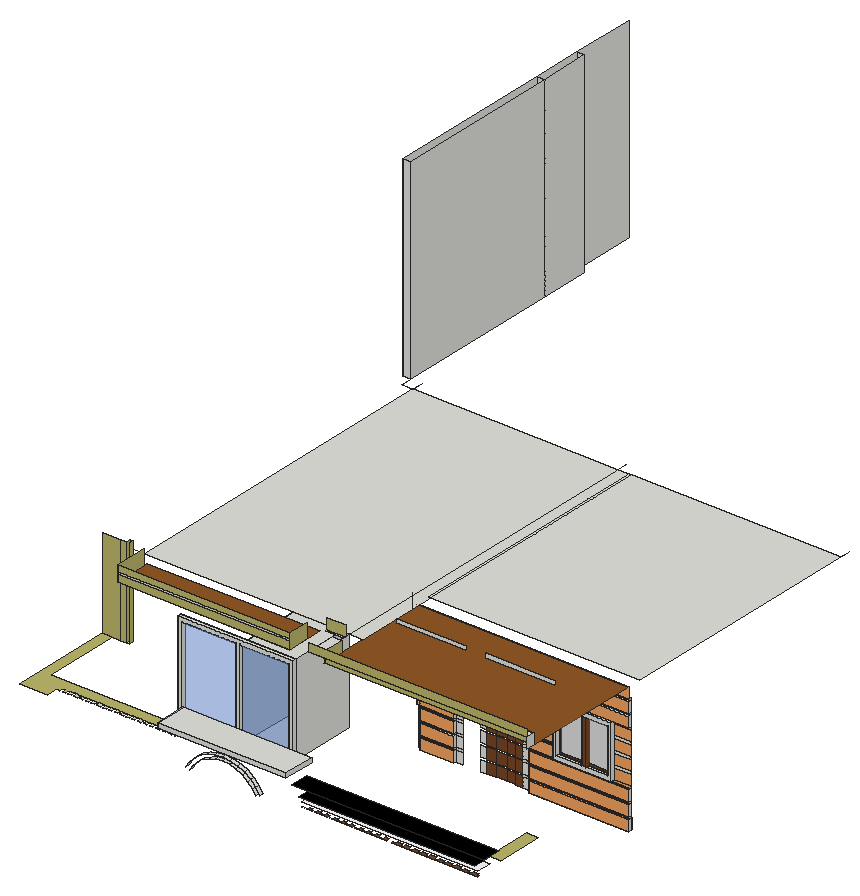
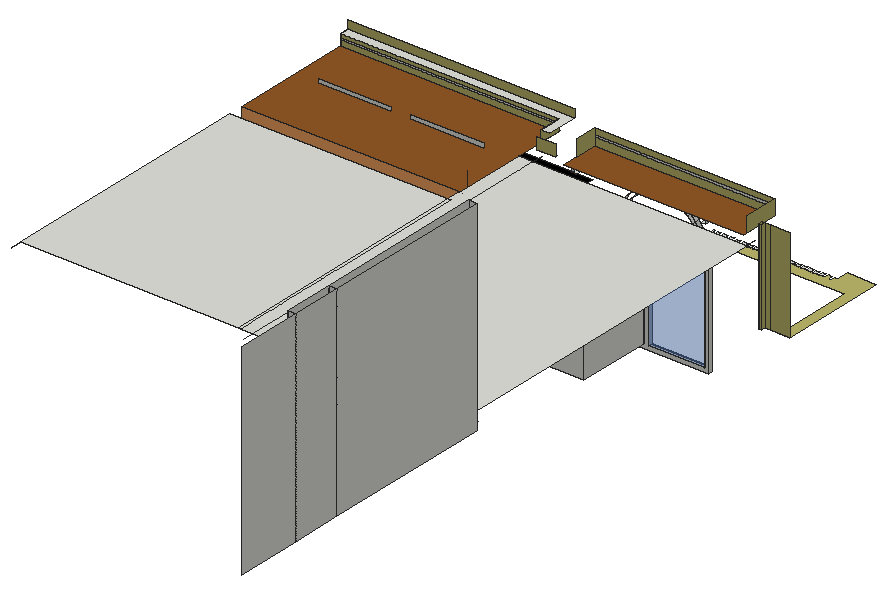
# SketchUp Ruby script. Lengths in inches.
U = 1.inch
M = Sketchup.active_model
def pt(a) = Geom::Point3d.new(a.map { |v| v * U })
def face(e, loops, mat)
  f = e.add_face(loops[0].map { |a| pt(a) })
  loops[1..].each { |l| e.add_face(l.map { |a| pt(a) }).erase! }
  f.material = f.back_material = mat if mat
  f
end
# faces: each face lists its corners as indices into pts; further lists are holes
def faces(e, pts, list, mat = nil) = list.each { |f| face(e, (f[0].is_a?(Array) ? f : [f]).map { |l| l.map { |i| pts[i] } }, mat) }
# xy, xz, yz: faces in a plane at the given z, y or x. An outline is a flat list of corners, or four numbers for a rectangle; further outlines are holes
def ring(l) = l.size == 4 ? [[l[0], l[1]], [l[2], l[1]], [l[2], l[3]], [l[0], l[3]]] : l.each_slice(2).to_a
def flat(e, list, mat, &to3) = list.each { |f| face(e, (f[0].is_a?(Array) ? f : [f]).map { |l| ring(l).map { |u, v| to3.(u, v) } }, mat) }
def xy(e, z, list, mat = nil) = flat(e, list, mat) { |x, y| [x, y, z] }
def xz(e, y, list, mat = nil) = flat(e, list, mat) { |x, z| [x, y, z] }
def yz(e, x, list, mat = nil) = flat(e, list, mat) { |y, z| [x, y, z] }
def lines(e, pts, list) = list.each { |a, b| e.add_line(pt(pts[a]), pt(pts[b])) }
# prism: a flat outline (further loops are holes) pulled along v
def prism(e, loops, v, mat = nil)
  f = face(e, loops, mat); d = Geom::Vector3d.new(v.map { |x| x * U })
  f.pushpull(f.normal.samedirection?(d) ? d.length : -d.length)
end
def box(e, o, s, mat = nil) = prism(e, [[o, [o[0] + s[0], o[1], o[2]], [o[0] + s[0], o[1] + s[1], o[2]], [o[0], o[1] + s[1], o[2]]]], [0, 0, s[2]], mat)
def at(x, y, z, deg = 0) = Geom::Transformation.translation(pt([x, y, z])) * Geom::Transformation.rotation(ORIGIN, Z_AXIS, deg.degrees)
def axes(o, x, y, z) = Geom::Transformation.new([*x, 0, *y, 0, *z, 0, *pt(o).to_a, 1])
def part(name) = M.definitions.add(name)
# library, detail: a bought-in or finely detailed component or shape, given as its bounding box
def library(name, o, s) = part(name).tap { |d| box(d.entities, o, s) }
def detail(e, o, s) = box(e.add_group.entities, o, s)
def put(e, d, t, mat = nil) = e.add_instance(d, t).tap { |i| i.material = mat if mat }
def group(e, t, mat = nil) = e.add_group.tap { |g| g.transformation = t; g.material = mat if mat }.entities
root = M.entities
M.materials.add("[0010_Snow]").color = [255, 250, 250]
M.materials.add("[0037_SandyBrown]").color = [244, 164, 96]
M.materials.add("[0057_DarkKhaki]").color = [189, 183, 107]
M.materials.add("[0137_Black]").color = [0, 0, 0]
M.materials.add("[Translucent Glass Blue]").color = [100, 149, 237]
M.materials["[Translucent Glass Blue]"].alpha = 0.5
M.materials.add("[Translucent Glass Gray]").color = [128, 128, 128]
M.materials["[Translucent Glass Gray]"].alpha = 0.5
M.materials.add("[Wood Floor Parquet]").color = [145, 89, 39]
M.materials.add("[Wood Veneer 01]").color = [120, 70, 37]
xy(root,15.35,[[88.6875,87.625,180.5,90.625]])
xy(root,16.53,[[227.125,155.75,254.53,157.75],[314.53,155.75,394.3125,157.75],[314.53,157.75,394.3125,158.9375]])
xy(root,18.35,[[91.6875,87.625,134.59,90.625],[138.39,87.625,177.5,90.625],[138.39,90.625,177.5,147.4375]])
xy(root,24.9375,[[314.53,157.75,394.3125,158.9375]])
xy(root,24.9375,[[227.125,155.75,254.53,157.75],[314.53,155.75,394.3125,157.75]],"[0037_SandyBrown]")
xy(root,27.1,[[227.125,155.75,254.53,157.75],[314.53,155.75,394.3125,157.75]])
xy(root,35.5,[[227.125,155.75,254.53,157.75]])
xy(root,35.5,[[314.53,155.75,394.3125,157.75]],"[0037_SandyBrown]")
xy(root,37.66,[[227.125,155.75,254.53,157.75],[314.53,155.75,394.3125,157.75]])
xy(root,44.24,[[246.54,13.8125,246.54,14.8125,250.6,14.8125,250.6,16.8125,253.29,16.8125,253.29,14.8125,257.35,14.8125,257.35,16.8125,260.04,16.8125,260.04,14.8125,264.1,14.8125,264.1,16.8125,266.79,16.8125,266.79,14.8125,270.85,14.8125,270.85,16.8125,273.54,16.8125,273.54,14.8125,277.6,14.8125,277.6,16.8125,280.29,16.8125,280.29,14.8125,284.35,14.8125,284.35,16.8125,287.04,16.8125,287.04,14.8125,291.1,14.8125,291.1,16.8125,293.79,16.8125,293.79,14.8125,297.85,14.8125,297.85,16.8125,300.54,16.8125,300.54,14.8125,304.6,14.8125,304.6,16.8125,307.29,16.8125,307.29,14.8125,311.35,14.8125,311.35,16.8125,314.04,16.8125,314.04,14.8125,314.71,14.8125,314.71,13.8125],[318.91,13.8125,318.91,14.8125,320.79,14.8125,320.79,16.8125,324.85,16.8125,324.85,14.8125,327.54,14.8125,327.54,16.8125,331.6,16.8125,331.6,14.8125,334.29,14.8125,334.29,16.8125,338.35,16.8125,338.35,14.8125,341.04,14.8125,341.04,16.8125,345.1,16.8125,345.1,14.8125,347.79,14.8125,347.79,16.8125,351.85,16.8125,351.85,14.8125,354.54,14.8125,354.54,16.8125,358.6,16.8125,358.6,14.8125,361.29,14.8125,361.29,16.8125,365.35,16.8125,365.35,14.8125,368.04,14.8125,368.04,16.8125,372.1,16.8125,372.1,14.8125,374.79,14.8125,374.79,16.8125,378.85,16.8125,378.85,14.8125,381.54,14.8125,381.54,16.8125,385.6,16.8125,385.6,14.8125,387.24,14.8125,387.24,13.8125]],"[Wood Veneer 01]")
xy(root,46.0625,[[227.125,155.75,254.53,157.75],[314.53,155.75,394.3125,157.75]])
xy(root,48.04,[[334.36,154.75,381.24,157.75]])
xy(root,48.11,[[246.54,13.8125,387.24,25.8125]],"[0010_Snow]")
xy(root,48.22,[[225.0625,155.75,227.125,157.75],[227.125,155.75,254.53,157.75],[314.53,155.75,334.36,157.75]])
xy(root,51.04,[[337.36,154.75,357.8,157.75],[360.74,154.75,378.24,157.75]])
xy(root,53.24,[[246.54,10.8125,387.24,25.8125]],"[0137_Black]")
xy(root,56.625,[[225.0625,155.75,227.125,157.75],[227.125,155.75,254.53,157.75],[314.53,155.75,334.36,157.75]])
xy(root,58.78,[[225.0625,155.75,227.125,157.75],[227.125,155.75,254.53,157.75],[314.53,155.75,334.36,157.75]])
xy(root,60,[[59.94,13.8125,62.74,16.8125],[64.57,13.8125,67.37,16.8125],[69.19,13.8125,71.99,16.8125],[73.82,13.8125,76.62,16.8125],[78.44,13.8125,81.24,16.8125],
  [83.07,13.8125,85.87,16.8125],[87.69,13.8125,90.49,16.8125],[92.32,13.8125,95.12,16.8125],[96.94,13.8125,99.74,16.8125],[101.57,13.8125,104.37,16.8125],
  [106.19,13.8125,108.99,16.8125],[110.82,13.8125,113.62,16.8125],[115.44,13.8125,118.24,16.8125],[120.07,13.8125,122.87,16.8125],[125.13,13.8125,127.93,16.8125],
  [130.19,13.8125,132.99,16.8125],[135.25,13.8125,138.06,16.8125],[140.32,13.8125,143.12,16.8125],[145.38,13.8125,145.98,16.8125],[47.8125,87.625,50.0625,90.625]])
xy(root,60,[[28.5625,4.8125,50.69,4.8125,50.69,13.8125,53.49,13.8125,53.49,16.8125,55.32,16.8125,55.32,13.8125,58.12,13.8125,58.12,16.8125,145.98,16.8125,145.98,25.8125,36.25,25.8125,36.25,87.625,28.5625,87.625],[394.3125,16.8125,403.3125,54.1875]],"[0057_DarkKhaki]")
xy(root,60,[[241.27,10.8125,394.3125,25.8125]],"[0137_Black]")
xy(root,67.1875,[[225.0625,155.75,227.125,157.75],[227.125,155.75,254.53,157.75],[314.53,155.75,334.36,157.75]])
xy(root,69.35,[[225.0625,155.75,227.125,157.75],[227.125,155.75,254.53,157.75],[314.53,155.75,334.36,157.75],[225.0625,157.75,254.53,157.875]])
xy(root,70.61,[[142.42,0,142.42,25.8125,145.98,25.8125,145.98,4.8125,241.27,4.8125,241.27,25.8125,244.96,25.8125,244.96,0]])
xy(root,74.1875,[[142.42,0,244.96,25.8125]])
xy(root,77.75,[[225.0625,155.75,227.125,157.75],[314.53,155.75,334.36,157.75],[225.0625,157.75,254.53,157.875]])
xy(root,77.75,[[227.125,155.75,254.53,157.75]],"[0037_SandyBrown]")
xy(root,79.91,[[225.0625,155.75,227.125,157.75],[227.125,155.75,254.53,157.75],[314.53,155.75,334.36,157.75]])
xy(root,84,[[260.53,154.75,274.66,157.75],[274.66,154.75,279.73,157.75],[279.73,154.75,308.53,157.75]])
xy(root,87.22,[[337.36,154.75,357.8,157.75],[360.74,154.75,378.24,157.75]])
xy(root,88.3125,[[225.0625,155.75,227.125,157.75],[227.125,155.75,254.53,157.75],[314.53,155.75,334.36,157.75]])
xy(root,90,[[254.53,154.75,314.53,157.75]])
xy(root,90.22,[[334.36,154.75,381.24,157.75]])
xy(root,90.47,[[225.0625,155.75,227.125,157.75],[227.125,155.75,394.3125,157.75]])
xy(root,90.6,[[91.6875,87.625,134.59,90.625],[134.59,87.625,138.39,90.625],[138.39,87.625,177.5,90.625],[138.39,90.625,177.5,147.4375]])
xy(root,93.6,[[88.6875,87.625,180.5,90.625]])
xy(root,98.875,[[225.0625,155.75,227.125,157.75],[227.125,155.75,394.3125,157.75]])
xy(root,101.03,[[225.0625,155.75,227.125,157.75],[227.125,155.75,394.3125,157.75]])
xy(root,109.4375,[[225.0625,155.75,227.125,157.75],[227.125,155.75,394.3125,157.75]])
xy(root,111.6,[[225.0625,155.75,227.125,157.75],[227.125,155.75,394.3125,157.75]])
xy(root,120,[[52.3125,99.625,216.0625,367.8125],[216.0625,99.625,216.0625,367.8125,225.0625,367.8125,225.0625,166.75,227.125,166.75,227.125,99.625],[225.0625,166.75,227.125,367.8125],[227.125,166.75,394.3125,367.8125],[37.25,376.8125,43.3125,510.5],
  [37.25,510.5,43.3125,550.125]])
xy(root,120,[[61.7,61.0625,199.44,90.625],[227.125,61.0625,394.3125,155.75]],"[Wood Floor Parquet]")
xy(root,123.17,[[205.65,89.5625,220.06,90.625]])
xy(root,128.6875,[[220.06,54.1875,220.06,77.875,227.125,77.875,227.125,61.0625,394.3125,61.0625,394.3125,54.1875]])
xz(root,0,[[142.42,70.61,244.96,74.1875]])
xz(root,25.8125,[[241.27,70.61,244.96,70.75]])
xz(root,54.1875,[[220.06,128.6875,394.3125,134.75]],"[0057_DarkKhaki]")
xz(root,61.0625,[[227.125,124.34,394.3125,125.71],[61.7,126,199.44,127.5]])
xz(root,61.0625,[[61.7,120,199.44,126],[227.125,120,394.3125,124.34],[227.125,125.71,394.3125,128.6875],[61.7,127.5,199.44,132]],"[0057_DarkKhaki]")
xz(root,87.625,[[[88.6875,15.35,180.5,93.6],[91.6875,18.35,91.6875,90.6,177.5,90.6,177.5,18.35,138.39,18.35,138.39,90.6,134.59,90.6,134.59,18.35]]])
xz(root,87.625,[[28.5625,60,43.3125,132],[43.3125,60,47.8125,132]],"[0057_DarkKhaki]")
xz(root,90.625,[[[88.6875,15.35,180.5,93.6],[91.6875,18.35,134.59,18.35,134.59,90.6,138.39,90.6,138.39,18.35,177.5,18.35,177.5,90.6,91.6875,90.6]]])
xz(root,90.625,[[47.8125,60,50.0625,132],[205.65,123.17,220.06,132]],"[0057_DarkKhaki]")
xz(root,90.625,[[91.6875,18.35,134.59,90.6],[138.39,18.35,177.5,90.6]],"[Translucent Glass Blue]")
xz(root,116.875,[[239.99,129,295.56,132],[310.99,129,366.56,132]])
xz(root,147.4375,[[138.39,18.35,177.5,90.6]])
xz(root,154.75,[[[334.36,48.04,381.24,90.22],[337.36,51.04,378.24,87.22]]])
xz(root,154.75,[[357.8,51.04,360.74,87.22]],"[Wood Veneer 01]")
xz(root,155.75,[[225.0625,48.22,227.125,56.625],[225.0625,58.78,227.125,67.1875],[225.0625,69.35,227.125,77.75],[225.0625,79.91,227.125,88.3125],[225.0625,90.47,227.125,98.875],
  [225.0625,101.03,227.125,109.4375]])
xz(root,155.75,[[227.125,16.53,254.53,24.9375],[314.53,16.53,394.3125,24.9375],[227.125,27.1,254.53,35.5],[314.53,27.1,394.3125,35.5],[227.125,37.66,254.53,46.0625],
  [314.53,37.66,394.3125,46.0625],[227.125,48.22,254.53,56.625],[314.53,48.22,334.36,56.625],[227.125,58.78,254.53,67.1875],[314.53,58.78,334.36,67.1875],
  [227.125,69.35,254.53,77.75],[314.53,69.35,334.36,77.75],[227.125,79.91,254.53,88.3125],[314.53,79.91,334.36,88.3125],[227.125,90.47,394.3125,98.875],
  [227.125,101.03,394.3125,109.4375],[227.125,111.6,394.3125,120]],"[0037_SandyBrown]")
xz(root,157.75,[[225.0625,16.53,227.125,24.9375],[227.125,16.53,254.53,24.9375],[254.53,16.53,260.53,24.9375],[274.66,16.53,279.73,24.9375],[308.53,16.53,314.53,24.9375],
  [314.53,16.53,394.3125,24.9375],[225.0625,24.9375,227.125,27.1],[254.53,24.9375,260.53,27.1],[308.53,24.9375,314.53,27.1],[225.0625,27.1,227.125,35.5],
  [227.125,27.1,254.53,35.5],[254.53,27.1,260.53,35.5],[274.66,27.1,279.73,35.5],[308.53,27.1,314.53,35.5],[314.53,27.1,394.3125,35.5],
  [225.0625,35.5,227.125,37.66],[254.53,35.5,260.53,37.66],[308.53,35.5,314.53,37.66],[225.0625,37.66,227.125,46.0625],[254.53,37.66,260.53,46.0625],
  [274.66,37.66,279.73,46.0625],[308.53,37.66,314.53,46.0625],[314.53,37.66,394.3125,46.0625],[225.0625,46.0625,227.125,48.22],[254.53,46.0625,260.53,48.22],
  [308.53,46.0625,314.53,48.22],[334.36,48.04,381.24,48.22],[225.0625,48.22,254.53,56.625],[254.53,48.22,260.53,56.625],[274.66,48.22,279.73,56.625],
  [308.53,48.22,314.53,56.625],[314.53,48.22,334.36,56.625],[334.36,48.22,381.24,48.22,381.24,56.625,378.24,56.625,378.24,51.04,360.74,51.04,360.74,52.68,357.8,52.68,357.8,51.04,337.36,51.04,337.36,56.625,334.36,56.625],[357.8,52.68,360.74,56.625],[225.0625,56.625,227.125,58.78],
  [254.53,56.625,260.53,58.78],[308.53,56.625,314.53,58.78],[334.36,56.625,337.36,58.78],[357.8,56.625,360.74,58.78],[378.24,56.625,381.24,58.78],
  [381.24,56.625,394.3125,58.78],[225.0625,58.78,254.53,67.1875],[254.53,58.78,260.53,67.1875],[274.66,58.78,279.73,67.1875],[308.53,58.78,314.53,67.1875],
  [314.53,58.78,334.36,67.1875],[334.36,58.78,337.36,67.1875],[357.8,58.78,360.74,67.1875],[378.24,58.78,381.24,67.1875],[225.0625,67.1875,227.125,69.35],
  [254.53,67.1875,260.53,69.35],[308.53,67.1875,314.53,69.35],[334.36,67.1875,337.36,69.35],[357.8,67.1875,360.74,69.35],[378.24,67.1875,381.24,69.35],
  [381.24,67.1875,394.3125,69.35],[225.0625,69.35,254.53,77.75],[254.53,69.35,260.53,77.75],[274.66,69.35,279.73,77.75],[308.53,69.35,314.53,77.75],
  [334.36,69.35,337.36,77.75],[357.8,69.35,360.74,77.75],[378.24,69.35,381.24,77.75],[225.0625,77.75,227.125,79.91],[254.53,77.75,260.53,79.91],
  [308.53,77.75,314.53,79.91],[334.36,77.75,337.36,79.91],[357.8,77.75,360.74,79.91],[378.24,77.75,381.24,79.91],[381.24,77.75,394.3125,79.91],
  [225.0625,79.91,254.53,88.3125],[254.53,79.91,260.53,79.91,260.53,84,308.53,84,308.53,79.91,314.53,79.91,314.53,88.3125,254.53,88.3125],[274.66,79.91,279.73,84],[334.36,79.91,337.36,79.91,337.36,87.22,357.8,87.22,357.8,85.75,360.74,85.75,360.74,87.22,378.24,87.22,378.24,79.91,381.24,79.91,381.24,88.3125,334.36,88.3125],[357.8,79.91,360.74,85.75],
  [225.0625,88.3125,227.125,90.47],[254.53,88.3125,314.53,90],[334.36,88.3125,381.24,90.22],[225.0625,90.47,394.3125,98.875],[225.0625,98.875,227.125,101.03],
  [225.0625,101.03,394.3125,109.4375],[225.0625,109.4375,227.125,111.6]])
xz(root,157.75,[[227.125,24.9375,254.53,27.1],[314.53,24.9375,394.3125,27.1],[227.125,35.5,254.53,37.66],[314.53,35.5,394.3125,37.66],[227.125,46.0625,254.53,48.22],
  [314.53,46.0625,394.3125,46.0625,394.3125,48.22,381.24,48.22,381.24,48.04,334.36,48.04,334.36,48.22,314.53,48.22],[381.24,48.22,394.3125,56.625],[227.125,56.625,254.53,58.78],[314.53,56.625,334.36,58.78],[381.24,58.78,394.3125,67.1875],
  [227.125,67.1875,254.53,69.35],[314.53,67.1875,334.36,69.35],[381.24,69.35,394.3125,77.75],[227.125,77.75,254.53,79.91],[314.53,77.75,334.36,79.91],
  [381.24,79.91,394.3125,88.3125],[227.125,88.3125,254.53,88.3125,254.53,90,314.53,90,314.53,88.3125,334.36,88.3125,334.36,90.22,381.24,90.22,381.24,88.3125,394.3125,88.3125,394.3125,90.47,227.125,90.47],[227.125,98.875,394.3125,101.03],[227.125,109.4375,394.3125,111.6]],"[0037_SandyBrown]")
xz(root,157.75,[[338.85,52.68,357.8,85.75],[360.74,52.68,377.24,85.75]],"[Translucent Glass Gray]")
xz(root,157.75,[[279.73,17.03,286.72,25.59],[287.41,17.03,295.09,25.59],[295.95,17.03,302.05,25.59],[302.96,17.03,308.53,25.59],[279.73,26.78,286.72,35.97],
  [287.41,26.78,295.09,35.97],[295.95,26.78,302.05,35.97],[302.96,26.78,308.53,35.97],[279.73,37.15,286.72,46.34],[287.41,37.15,295.09,46.34],
  [295.95,37.15,302.05,46.34],[302.96,37.15,308.53,46.34],[279.73,47.53,286.72,56.72],[287.41,47.53,295.09,56.72],[295.95,47.53,302.05,56.72],
  [302.96,47.53,308.53,56.72],[337.36,51.04,357.8,51.04,357.8,52.68,338.85,52.68,338.85,85.75,357.8,85.75,357.8,87.22,337.36,87.22],[360.74,51.04,378.24,51.04,378.24,87.22,360.74,87.22,360.74,85.75,377.24,85.75,377.24,52.68,360.74,52.68],[279.73,57.9,286.72,67.09],[287.41,57.9,295.09,67.09],
  [295.95,57.9,302.05,67.09],[302.96,57.9,308.53,67.09],[279.73,68.28,286.72,77.47],[287.41,68.28,295.09,77.47],[295.95,68.28,302.05,77.47],
  [302.96,68.28,308.53,77.47],[279.73,78.65,286.72,84],[287.41,78.65,295.09,84],[295.95,78.65,302.05,84],[302.96,78.65,308.53,84]],"[Wood Veneer 01]")
xz(root,157.875,[[225.0625,69.35,254.53,77.75]])
xz(root,158.9375,[[314.53,16.53,394.3125,24.9375]])
xz(root,376.8125,[[37.25,120,43.3125,276]])
xz(root,510.5,[[37.25,120,43.3125,276]])
xz(root,550.125,[[37.25,120,43.3125,276]])
yz(root,37.25,[[376.8125,120,510.5,276],[510.5,120,550.125,276],[550.125,120,601.9375,276]])
yz(root,43.3125,[[376.8125,120,510.5,276],[510.5,120,550.125,276]])
yz(root,47.8125,[[87.625,60,90.625,132]],"[0057_DarkKhaki]")
yz(root,50.0625,[[87.625,60,90.625,132]],"[0057_DarkKhaki]")
yz(root,61.7,[[61.0625,120,87.625,132]],"[0057_DarkKhaki]")
yz(root,88.6875,[[87.625,15.35,90.625,93.6]])
yz(root,91.6875,[[87.625,18.35,90.625,90.6]])
yz(root,134.59,[[87.625,18.35,90.625,90.6]])
yz(root,138.39,[[87.625,18.35,90.625,90.6],[90.625,18.35,147.4375,90.6]])
yz(root,142.42,[[0,70.61,25.8125,74.1875]])
yz(root,177.5,[[87.625,18.35,90.625,90.6],[90.625,18.35,147.4375,90.6]])
yz(root,180.5,[[87.625,15.35,90.625,93.6]])
yz(root,199.44,[[61.0625,120,77.875,132]],"[0057_DarkKhaki]")
yz(root,225.0625,[[155.75,48.22,157.75,56.625],[155.75,58.78,157.75,67.1875],[155.75,69.35,157.75,77.75],[157.75,69.35,157.875,77.75],[155.75,79.91,157.75,88.3125],
  [155.75,90.47,157.75,98.875],[155.75,101.03,157.75,109.4375]])
yz(root,227.125,[[155.75,16.53,157.75,24.9375],[155.75,27.1,157.75,35.5],[155.75,37.66,157.75,46.0625]])
yz(root,227.125,[[61.0625,120,77.875,128.6875]],"[0057_DarkKhaki]")
yz(root,244.96,[[0,70.61,25.8125,74.1875]])
yz(root,254.53,[[155.75,16.53,157.75,24.9375],[155.75,27.1,157.75,35.5],[155.75,37.66,157.75,46.0625],[155.75,48.22,157.75,56.625],[155.75,58.78,157.75,67.1875],
  [155.75,69.35,157.75,77.75],[157.75,69.35,157.875,77.75],[155.75,79.91,157.75,88.3125]])
yz(root,314.53,[[155.75,16.53,157.75,24.9375],[157.75,16.53,158.9375,24.9375],[155.75,27.1,157.75,35.5],[155.75,37.66,157.75,46.0625],[155.75,48.22,157.75,56.625],
  [155.75,58.78,157.75,67.1875],[155.75,69.35,157.75,77.75],[155.75,79.91,157.75,88.3125]])
yz(root,334.36,[[154.75,48.04,154.75,90.22,157.75,90.22,157.75,88.3125,155.75,88.3125,155.75,79.91,157.75,79.91,157.75,77.75,155.75,77.75,155.75,69.35,157.75,69.35,157.75,67.1875,155.75,67.1875,155.75,58.78,157.75,58.78,157.75,56.625,155.75,56.625,155.75,48.22,157.75,48.22,157.75,48.04],[155.75,48.22,157.75,56.625],[155.75,58.78,157.75,67.1875],[155.75,69.35,157.75,77.75],[155.75,79.91,157.75,88.3125]])
yz(root,337.36,[[154.75,51.04,157.75,87.22]])
yz(root,357.8,[[154.75,51.04,157.75,87.22]],"[Wood Veneer 01]")
yz(root,360.74,[[154.75,51.04,157.75,87.22]],"[Wood Veneer 01]")
yz(root,378.24,[[154.75,51.04,157.75,87.22]])
yz(root,381.24,[[154.75,48.04,157.75,90.22]])
yz(root,394.3125,[[155.75,16.53,157.75,24.9375],[157.75,16.53,158.9375,24.9375],[155.75,27.1,157.75,35.5],[155.75,37.66,157.75,46.0625],[155.75,90.47,157.75,98.875],
  [155.75,101.03,157.75,109.4375],[54.1875,120,61.0625,128.6875]])
p = [[166.64,4.8125,48.36],[169.3,4.8125,52.43],[169.3,1.8125,52.43],[166.64,1.8125,48.36],[217.05,4.8125,52.43],[219.7,4.8125,48.36],
  [219.7,1.8125,48.36],[217.05,1.8125,52.43],[166.93,4.8125,54.29],[163.64,4.8125,49.25],[163.64,1.8125,49.25],[166.93,1.8125,54.29],
  [222.7,4.8125,49.25],[219.41,4.8125,54.29],[219.41,1.8125,54.29],[222.7,1.8125,49.25],[173.07,4.8125,56.4],[173.07,1.8125,56.4],
  [213.27,4.8125,56.4],[213.27,1.8125,56.4],[171.08,4.8125,58.67],[171.08,1.8125,58.67],[215.26,4.8125,58.67],[215.26,1.8125,58.67],
  [177.5,4.8125,59.64],[177.5,1.8125,59.64],[208.85,4.8125,59.64],[208.85,1.8125,59.64],[175.94,4.8125,62.22],[175.94,1.8125,62.22],
  [210.4,4.8125,62.22],[210.4,1.8125,62.22],[182.43,4.8125,62.03],[182.43,1.8125,62.03],[203.91,4.8125,62.03],[203.91,1.8125,62.03],
  [187.71,4.8125,63.5],[187.71,1.8125,63.5],[198.63,4.8125,63.5],[198.63,1.8125,63.5],[181.37,4.8125,64.85],[181.37,1.8125,64.85],
  [204.98,4.8125,64.85],[204.98,1.8125,64.85],[193.17,4.8125,63.99],[193.17,1.8125,63.99],[187.17,4.8125,66.46],[187.17,1.8125,66.46],
  [199.17,4.8125,66.46],[199.17,1.8125,66.46],[193.17,4.8125,67],[193.17,1.8125,67],[225.0625,155.75,111.6],[225.0625,155.75,120],
  [216.0625,99.625,120],[216.0625,90.625,120],[52.3125,99.625,120],[52.3125,90.625,120],[52.3125,367.8125,120],[43.3125,367.8125,120],
  [43.3125,99.625,120],[52.3125,376.8125,120],[394.3125,367.8125,120],[394.3125,376.8125,120],[216.0625,367.8125,120],[216.0625,376.8125,120],
  [227.125,61.0625,120],[227.125,59.84,120],[227.125,148.375,132],[227.125,148.375,120],[43.3125,376.8125,120]]
faces(root,p,[[0,1,2,3],[4,5,6,7],[8,9,10,11],[12,13,14,15],[1,16,17,2],[18,4,7,19],[20,8,11,21],[13,22,23,14],
  [16,24,25,17],[26,18,19,27],[28,20,21,29],[22,30,31,23],[24,32,33,25],[34,26,27,35],[32,36,37,33],[38,34,35,39],
  [40,28,29,41],[30,42,43,31],[36,44,45,37],[44,38,39,45],[46,40,41,47],[42,48,49,43],[50,46,47,51],[48,50,51,49]])
lines(root,p,[[52,53],[54,55],[56,57],[58,59],[56,60],[58,61],[62,63],[64,65],[66,67],[68,69],[59,70]])
